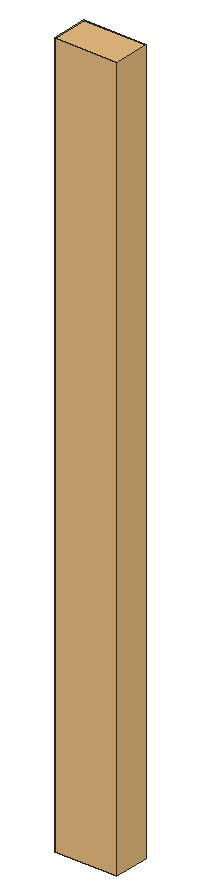
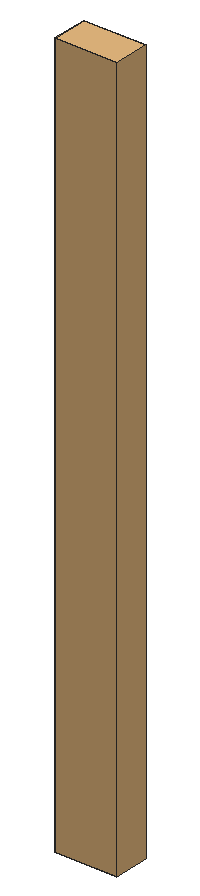
# SketchUp Ruby script. Lengths in inches.
U = 1.inch
M = Sketchup.active_model
def pt(a) = Geom::Point3d.new(a.map { |v| v * U })
def face(e, loops, mat)
  f = e.add_face(loops[0].map { |a| pt(a) })
  loops[1..].each { |l| e.add_face(l.map { |a| pt(a) }).erase! }
  f.material = f.back_material = mat if mat
  f
end
# faces: each face lists its corners as indices into pts; further lists are holes
def faces(e, pts, list, mat = nil) = list.each { |f| face(e, (f[0].is_a?(Array) ? f : [f]).map { |l| l.map { |i| pts[i] } }, mat) }
# xy, xz, yz: faces in a plane at the given z, y or x. An outline is a flat list of corners, or four numbers for a rectangle; further outlines are holes
def ring(l) = l.size == 4 ? [[l[0], l[1]], [l[2], l[1]], [l[2], l[3]], [l[0], l[3]]] : l.each_slice(2).to_a
def flat(e, list, mat, &to3) = list.each { |f| face(e, (f[0].is_a?(Array) ? f : [f]).map { |l| ring(l).map { |u, v| to3.(u, v) } }, mat) }
def xy(e, z, list, mat = nil) = flat(e, list, mat) { |x, y| [x, y, z] }
def xz(e, y, list, mat = nil) = flat(e, list, mat) { |x, z| [x, y, z] }
def yz(e, x, list, mat = nil) = flat(e, list, mat) { |y, z| [x, y, z] }
def lines(e, pts, list) = list.each { |a, b| e.add_line(pt(pts[a]), pt(pts[b])) }
# prism: a flat outline (further loops are holes) pulled along v
def prism(e, loops, v, mat = nil)
  f = face(e, loops, mat); d = Geom::Vector3d.new(v.map { |x| x * U })
  f.pushpull(f.normal.samedirection?(d) ? d.length : -d.length)
end
def box(e, o, s, mat = nil) = prism(e, [[o, [o[0] + s[0], o[1], o[2]], [o[0] + s[0], o[1] + s[1], o[2]], [o[0], o[1] + s[1], o[2]]]], [0, 0, s[2]], mat)
def at(x, y, z, deg = 0) = Geom::Transformation.translation(pt([x, y, z])) * Geom::Transformation.rotation(ORIGIN, Z_AXIS, deg.degrees)
def axes(o, x, y, z) = Geom::Transformation.new([*x, 0, *y, 0, *z, 0, *pt(o).to_a, 1])
def part(name) = M.definitions.add(name)
# library, detail: a bought-in or finely detailed component or shape, given as its bounding box
def library(name, o, s) = part(name).tap { |d| box(d.entities, o, s) }
def detail(e, o, s) = box(e.add_group.entities, o, s)
def put(e, d, t, mat = nil) = e.add_instance(d, t).tap { |i| i.material = mat if mat }
def group(e, t, mat = nil) = e.add_group.tap { |g| g.transformation = t; g.material = mat if mat }.entities
root = M.entities
c1 = library("sm2 y trunk",[0,0,0],[17.12,8.11,126.29])
put(root,c1,axes([67.19,93.58,10.53],[0.41205,0,0],[0,0.51153,0],[0,0,0.6557]))
